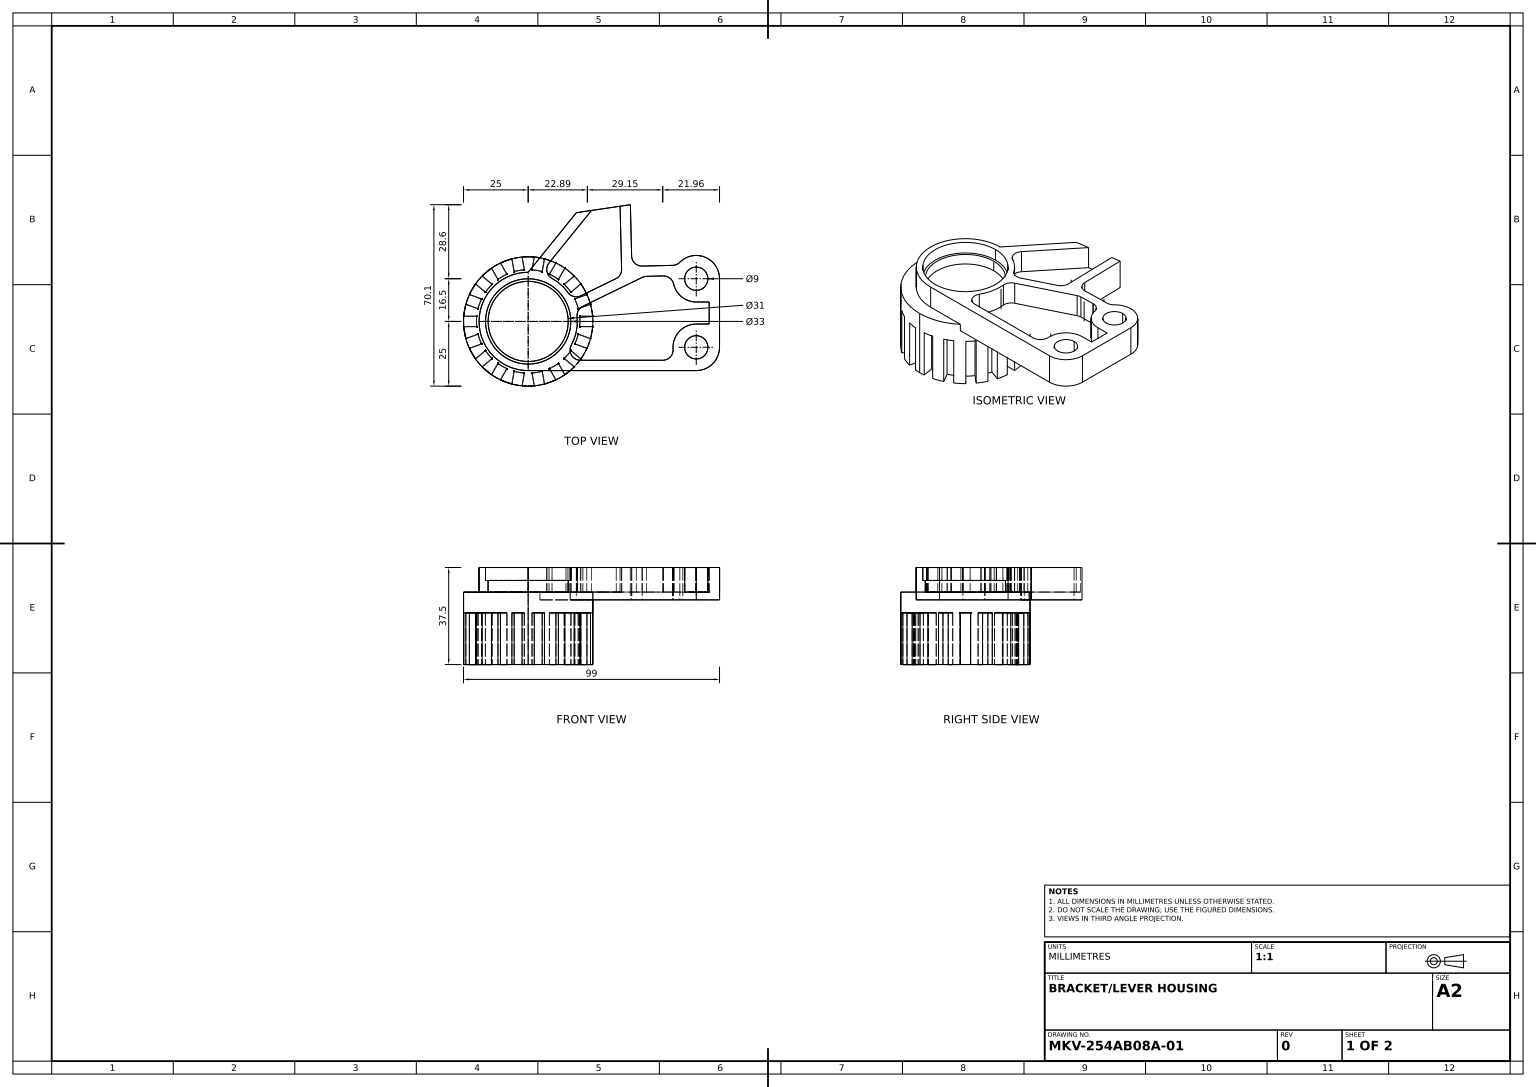
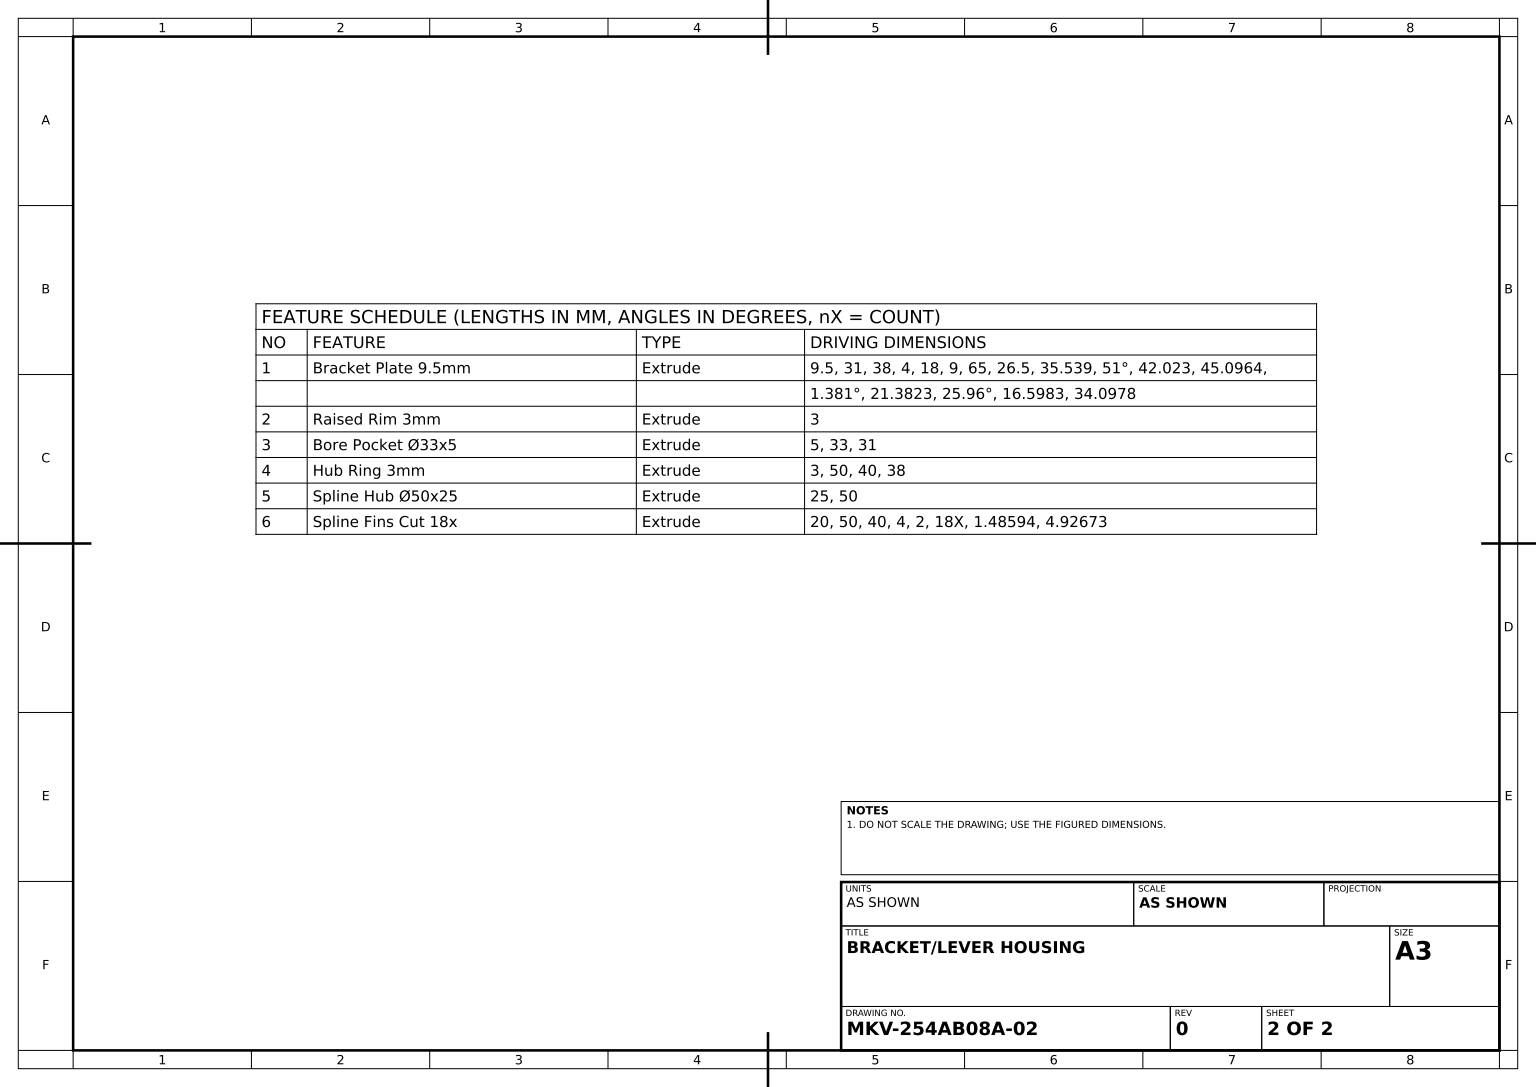
solid
v1 (65,0,14.5)
v2 (65,0,5.5)
e1 v1 v2 CIRCLE(AX(P(65,0,10),D(0,1,0),D(0,0,1)),4.5)
v3 (65,9.5,14.5)
e2 v3 v1 LINE
v4 (65,9.5,5.5)
e3 v3 v4 CIRCLE(AX(P(65,9.5,10),D(0,1,0),D(0,0,1)),4.5)
e4 v4 v2 LINE
face CYL(AX(P(65,9.5,10),D(0,-1,0),D(0,0,-1)),4.5) rev [-e1 -e2 e3 e4]
v5 (15.376876,9.5,-11.160273)
v6 (20.364842,9.5,-9.913285)
e5 v5 v6 CIRCLE(AX(P(18.614113,9.5,-13.509804),D(0,1,0),D(0,0,1)),4)
v7 (20.364842,0,-9.913285)
e6 v6 v7 LINE
v8 (15.376876,0,-11.160273)
e7 v8 v7 CIRCLE(AX(P(18.614113,0,-13.509804),D(0,1,0),D(0,0,1)),4)
e8 v5 v8 LINE
face CYL(AX(P(18.614113,9.5,-13.509804),D(0,-1,0),D(0,0,-1)),4) rev [e5 e6 -e7 -e8]
v9 (-19.899749,-28,-2)
v10 (-24.919872,-28,-2)
e9 v9 v10 LINE
v11 (-19.899749,-8,-2)
e10 v11 v9 LINE
v12 (-24.919872,-8,-2)
e11 v11 v12 LINE
e12 v12 v10 LINE
face PLANE(AX(P(0,-8,-2),D(0,0,1),D(1,0,0))) [-e9 -e10 e11 e12]
v13 (-1.48594,-8,19.944723)
v14 (-5.425171,-8,19.25013)
e13 v13 v14 CIRCLE(AX(P(0,-8,0),D(0,-1,0),D(0,0,-1)),20)
v15 (-5.425171,-28,19.25013)
e14 v14 v15 LINE
v16 (-1.48594,-28,19.944723)
e15 v16 v15 CIRCLE(AX(P(0,-28,0),D(0,-1,0),D(0,0,-1)),20)
e16 v13 v16 LINE
face CYL(AX(P(0,-8,0),D(0,-1,0),D(0,0,-1)),20) [e13 e14 -e15 -e16]
v17 (74,-3,-16.5)
v18 (74,-3,10)
e17 v17 v18 LINE
v19 (74,9.5,-16.5)
e18 v19 v17 LINE
v20 (74,9.5,10)
e19 v19 v20 LINE
e20 v20 v18 LINE
face PLANE(AX(P(74,9.5,0),D(1,0,0),D(0,0,-1))) [-e17 -e18 e19 e20]
v21 (-13.958517,-8,-14.323401)
v22 (-13.958517,-28,-14.323401)
e21 v21 v22 LINE
v23 (-16.529667,-28,-11.259223)
e22 v23 v22 CIRCLE(AX(P(0,-28,0),D(0,-1,0),D(0,0,-1)),20)
v24 (-16.529667,-8,-11.259223)
e23 v24 v23 LINE
e24 v24 v21 CIRCLE(AX(P(0,-8,0),D(0,-1,0),D(0,0,-1)),20)
face CYL(AX(P(0,-8,0),D(0,-1,0),D(0,0,-1)),20) [e21 -e22 -e23 e24]
v25 (52.236092,9.5,-17.577388)
v26 (52.236092,0,-17.577388)
e25 v25 v26 LINE
v27 (45.755023,9.5,-17.421109)
e26 v27 v25 LINE
v28 (45.755023,0,-17.421109)
e27 v27 v28 LINE
e28 v28 v26 LINE
face PLANE(AX(P(-0.393246,9.5,-16.308326),D(-0.024106198,0,-0.999709403),D(-0.999709403,0,0.024106198))) rev [-e25 -e26 e27 e28]
v29 (44.100719,9.5,-17.01879)
e29 v29 v27 CIRCLE(AX(P(45.851448,9.5,-13.422271),D(0,-1,0),D(0,0,1)),4)
v30 (44.100719,0,-17.01879)
e30 v29 v30 LINE
e31 v30 v28 CIRCLE(AX(P(45.851448,0,-13.422271),D(0,-1,0),D(0,0,1)),4)
face CYL(AX(P(45.851448,9.5,-13.422271),D(0,-1,0),D(0,0,-1)),4) rev [-e27 -e29 e30 e31]
v31 (36.125792,9.5,-20.175466)
v32 (36.125792,0,-20.175466)
e32 v31 v32 LINE
v33 (35.539017,9.5,-44.50962)
e33 v33 v31 LINE
v34 (35.539017,0,-44.50962)
e34 v33 v34 LINE
e35 v34 v32 LINE
face PLANE(AX(P(36.591011,9.5,-0.882327),D(0.999709403,0,-0.024106198),D(-0.024106198,0,-0.999709403))) rev [-e32 -e33 e34 e35]
v35 (11.681925,-8,-16.233688)
v36 (11.681925,-28,-16.233688)
e36 v35 v36 LINE
v37 (14.191987,-8,-20.581242)
e37 v35 v37 LINE
v38 (14.191987,-28,-20.581242)
e38 v37 v38 LINE
e39 v36 v38 LINE
face PLANE(AX(P(1.732051,-8,1),D(-0.866025404,0,-0.5),D(-0.5,0,0.866025404))) [-e36 e37 e38 -e39]
v39 (-17.804154,-8,-17.550274)
e40 v21 v39 LINE
v40 (-17.804154,-28,-17.550274)
e41 v39 v40 LINE
e42 v22 v40 LINE
face PLANE(AX(P(1.285575,-8,-1.532089),D(-0.64278761,0,0.766044443),D(0.766044443,0,0.64278761))) [-e21 e40 e41 -e42]
v41 (0,9.5,16.5)
v42 (0,9.5,-16.5)
e43 v41 v42 CIRCLE(AX(P(0,9.5,0),D(0,1,0),D(0,0,1)),16.5)
v43 (0,4.5,-16.5)
e44 v43 v42 LINE
v44 (0,4.5,16.5)
e45 v44 v43 CIRCLE(AX(P(0,4.5,0),D(0,1,0),D(0,0,1)),16.5)
e46 v44 v41 LINE
face CYL(AX(P(0,4.5,0),D(0,1,0),D(0,0,1)),16.5) rev [e43 -e44 -e45 e46]
v45 (1.48594,-8,-19.944723)
v46 (2.357675,-8,-24.888579)
e47 v45 v46 LINE
v47 (6.296906,-8,-24.193986)
e48 v46 v47 CIRCLE(AX(P(0,-8,0),D(0,-1,0),D(0,0,-1)),25)
v48 (5.425171,-8,-19.25013)
e49 v48 v47 LINE
e50 v45 v48 CIRCLE(AX(P(0,-8,0),D(0,-1,0),D(0,0,-1)),20)
face PLANE(AX(P(0,-8,0),D(0,-1,0),D(0,0,-1))) [e47 e48 -e49 -e50]
v49 (58.617258,9.5,-22.845125)
v50 (55.876909,9.5,-21.666343)
e51 v49 v50 CIRCLE(AX(P(55.780484,9.5,-25.66518),D(0,-1,0),D(0,0,1)),4)
v51 (58.617258,-3,-22.845125)
e52 v49 v51 LINE
v52 (55.876909,-3,-21.666343)
e53 v52 v51 CIRCLE(AX(P(55.780484,-3,-25.66518),D(0,1,0),D(0,0,-1)),4)
e54 v50 v52 LINE
face CYL(AX(P(55.780484,9.5,-25.66518),D(0,-1,0),D(0,0,-1)),4) rev [-e51 e52 -e53 -e54]
v53 (56.026667,9.5,10.692308)
v54 (56.026667,0,10.692308)
e55 v53 v54 LINE
v55 (65,9.5,1)
e56 v55 v53 CIRCLE(AX(P(65,9.5,10),D(0,1,0),D(0,0,1)),9)
v56 (65,0,1)
e57 v55 v56 LINE
e58 v56 v54 CIRCLE(AX(P(65,0,10),D(0,1,0),D(0,0,1)),9)
face CYL(AX(P(65,9.5,10),D(0,-1,0),D(0,0,-1)),9) [-e55 -e56 e57 e58]
v57 (-2.357675,-28,24.888579)
e59 v16 v57 LINE
v58 (-2.357675,-8,24.888579)
e60 v58 v57 LINE
e61 v13 v58 LINE
face PLANE(AX(P(1.969616,-8,0.347296),D(0.984807753,0,0.173648178),D(0.173648178,0,-0.984807753))) rev [e16 e59 -e60 -e61]
v59 (65,9.5,19)
v60 (65,-3,19)
e62 v59 v60 LINE
e63 v18 v60 CIRCLE(AX(P(65,-3,10),D(0,-1,0),D(0,0,-1)),9)
e64 v59 v20 CIRCLE(AX(P(65,9.5,10),D(0,1,0),D(0,0,1)),9)
face CYL(AX(P(65,9.5,10),D(0,-1,0),D(0,0,-1)),9) [e62 -e63 -e20 -e64]
v61 (19.899749,-8,2)
v62 (19.899749,-28,2)
e65 v61 v62 LINE
v63 (24.919872,-8,2)
e66 v61 v63 LINE
v64 (24.919872,-28,2)
e67 v63 v64 LINE
e68 v62 v64 LINE
face PLANE(AX(P(0,-8,2),D(0,0,-1),D(-1,0,0))) [-e65 e66 e67 -e68]
v65 (65,-3,-25.5)
e69 v65 v17 CIRCLE(AX(P(65,-3,-16.5),D(0,-1,0),D(0,0,-1)),9)
v66 (65,9.5,-25.5)
e70 v66 v65 LINE
e71 v19 v66 CIRCLE(AX(P(65,9.5,-16.5),D(0,1,0),D(0,0,1)),9)
face CYL(AX(P(65,9.5,-16.5),D(0,-1,0),D(0,0,-1)),9) [e18 -e69 -e70 -e71]
v67 (-18.015607,-8,8.6855)
v68 (-19.383687,-8,4.92673)
e72 v67 v68 CIRCLE(AX(P(0,-8,0),D(0,-1,0),D(0,0,-1)),20)
v69 (-22.732979,-8,10.402483)
e73 v67 v69 LINE
v70 (-24.10106,-8,6.643713)
e74 v69 v70 CIRCLE(AX(P(0,-8,0),D(0,-1,0),D(0,0,-1)),25)
e75 v68 v70 LINE
face PLANE(AX(P(0,-8,0),D(0,-1,0),D(0,0,-1))) [-e72 e73 e74 -e75]
v71 (-19.383687,-8,-4.92673)
v72 (-24.10106,-8,-6.643713)
e76 v71 v72 LINE
v73 (-22.732979,-8,-10.402483)
e77 v72 v73 CIRCLE(AX(P(0,-8,0),D(0,-1,0),D(0,0,-1)),25)
v74 (-18.015607,-8,-8.6855)
e78 v74 v73 LINE
e79 v71 v74 CIRCLE(AX(P(0,-8,0),D(0,-1,0),D(0,0,-1)),20)
face PLANE(AX(P(0,-8,0),D(0,-1,0),D(0,0,-1))) [e76 e77 -e78 -e79]
v75 (19.899749,-8,-2)
v76 (24.919872,-8,-2)
e80 v75 v76 LINE
e81 v76 v63 CIRCLE(AX(P(0,-8,0),D(0,-1,0),D(0,0,-1)),25)
e82 v75 v61 CIRCLE(AX(P(0,-8,0),D(0,-1,0),D(0,0,-1)),20)
face PLANE(AX(P(0,-8,0),D(0,-1,0),D(0,0,-1))) [e80 e81 -e66 -e82]
v77 (-13.958517,-8,14.323401)
v78 (-17.804154,-8,17.550274)
e83 v77 v78 LINE
v79 (-20.375304,-8,14.486096)
e84 v78 v79 CIRCLE(AX(P(0,-8,0),D(0,-1,0),D(0,0,-1)),25)
v80 (-16.529667,-8,11.259223)
e85 v80 v79 LINE
e86 v77 v80 CIRCLE(AX(P(0,-8,0),D(0,-1,0),D(0,0,-1)),20)
face PLANE(AX(P(0,-8,0),D(0,-1,0),D(0,0,-1))) [e83 e84 -e85 -e86]
v81 (-19.383687,-28,-4.92673)
v82 (-24.10106,-28,-6.643713)
e87 v81 v82 LINE
e88 v72 v82 LINE
e89 v71 v81 LINE
face PLANE(AX(P(-0.68404,-8,1.879385),D(-0.342020143,0,0.939692621),D(0.939692621,0,0.342020143))) rev [e87 -e88 -e76 e89]
v83 (-24.10106,-28,6.643713)
e90 v70 v83 LINE
v84 (-19.383687,-28,4.92673)
e91 v84 v83 LINE
e92 v68 v84 LINE
face PLANE(AX(P(-0.68404,-8,-1.879385),D(0.342020143,0,0.939692621),D(0.939692621,0,-0.342020143))) [e90 -e91 -e92 e75]
v85 (-22.732979,-28,10.402483)
e93 v69 v85 LINE
v86 (-18.015607,-28,8.6855)
e94 v67 v86 LINE
e95 v86 v85 LINE
face PLANE(AX(P(0.68404,-8,1.879385),D(0.342020143,0,0.939692621),D(0.939692621,0,-0.342020143))) rev [-e93 -e73 e94 e95]
v87 (20.19901,0,15)
v88 (52.038519,0,15)
e96 v87 v88 LINE
e97 v54 v88 CIRCLE(AX(P(52.038519,0,11),D(0,-1,0),D(0,0,1)),4)
v89 (70,0,1)
e98 v89 v56 LINE
v90 (70,0,-7.5)
e99 v90 v89 LINE
v91 (65,0,-7.5)
e100 v91 v90 LINE
v92 (56.230204,0,-14.477458)
e101 v92 v91 CIRCLE(AX(P(65,0,-16.5),D(0,1,0),D(0,0,1)),9)
v93 (52.332517,0,-17.578551)
e102 v93 v92 CIRCLE(AX(P(52.332517,0,-13.578551),D(0,-1,0),D(0,0,1)),4)
e103 v26 v93 CIRCLE(AX(P(52.332517,0,-13.578551),D(0,-1,0),D(0,0,1)),4)
v94 (21.139435,0,-5.841598)
e104 v94 v30 LINE
v95 (18.909266,0,-1.854631)
e105 v94 v95 CIRCLE(AX(P(22.890164,0,-2.245079),D(0,1,0),D(0,0,1)),4)
v96 (16.686139,0,9.086957)
e106 v96 v95 CIRCLE(AX(P(0,0,0),D(0,1,0),D(0,0,1)),19)
e107 v96 v87 CIRCLE(AX(P(20.19901,0,11),D(0,1,0),D(0,0,1)),4)
face PLANE(AX(P(0,0,0),D(0,-1,0),D(0,0,-1))) rev [e96 -e97 -e58 -e98 -e99 -e100 -e101 -e102 -e103 -e28 -e31 -e104 e105 -e106 e107]
v97 (21.139435,9.5,-5.841598)
e108 v97 v94 LINE
v98 (18.909266,9.5,-1.854631)
e109 v97 v98 CIRCLE(AX(P(22.890164,9.5,-2.245079),D(0,1,0),D(0,0,1)),4)
e110 v98 v95 LINE
face CYL(AX(P(22.890164,9.5,-2.245079),D(0,-1,0),D(0,0,-1)),4) rev [-e105 -e108 e109 e110]
v99 (20.375304,-8,-14.486096)
v100 (20.375304,-28,-14.486096)
e111 v99 v100 LINE
v101 (16.529667,-28,-11.259223)
e112 v101 v100 LINE
v102 (16.529667,-8,-11.259223)
e113 v102 v101 LINE
e114 v102 v99 LINE
face PLANE(AX(P(1.285575,-8,1.532089),D(-0.64278761,0,-0.766044443),D(-0.766044443,0,0.64278761))) [e111 -e112 -e113 e114]
v103 (65,9.5,-12)
v104 (65,0,-12)
e115 v103 v104 LINE
v105 (65,9.5,-21)
e116 v103 v105 CIRCLE(AX(P(65,9.5,-16.5),D(0,1,0),D(0,0,1)),4.5)
v106 (65,0,-21)
e117 v105 v106 LINE
e118 v104 v106 CIRCLE(AX(P(65,0,-16.5),D(0,1,0),D(0,0,1)),4.5)
face CYL(AX(P(65,9.5,-16.5),D(0,-1,0),D(0,0,-1)),4.5) rev [-e115 e116 e117 -e118]
e119 v86 v84 CIRCLE(AX(P(0,-28,0),D(0,-1,0),D(0,0,-1)),20)
face CYL(AX(P(0,-8,0),D(0,-1,0),D(0,0,-1)),20) [e92 -e119 -e94 e72]
v107 (-6.296906,-8,24.193986)
e120 v58 v107 CIRCLE(AX(P(0,-8,0),D(0,-1,0),D(0,0,-1)),25)
e121 v14 v107 LINE
face PLANE(AX(P(0,-8,0),D(0,-1,0),D(0,0,-1))) [e120 -e121 -e13 e61]
v108 (8.217824,-28,-18.233688)
v109 (10.727885,-28,-22.581242)
e122 v108 v109 LINE
v110 (10.727885,-8,-22.581242)
e123 v110 v109 LINE
v111 (8.217824,-8,-18.233688)
e124 v111 v110 LINE
e125 v111 v108 LINE
face PLANE(AX(P(-1.732051,-8,-1),D(-0.866025404,0,-0.5),D(-0.5,0,0.866025404))) rev [e122 -e123 -e124 e125]
v112 (-6.296906,-8,-24.193986)
v113 (-2.357675,-8,-24.888579)
e126 v112 v113 CIRCLE(AX(P(0,-8,0),D(0,-1,0),D(0,0,-1)),25)
v114 (-1.48594,-8,-19.944723)
e127 v114 v113 LINE
v115 (-5.425171,-8,-19.25013)
e128 v115 v114 CIRCLE(AX(P(0,-8,0),D(0,-1,0),D(0,0,-1)),20)
e129 v115 v112 LINE
face PLANE(AX(P(0,-8,0),D(0,-1,0),D(0,0,-1))) [e126 -e127 -e128 e129]
v116 (5.425171,-8,19.25013)
v117 (5.425171,-28,19.25013)
e130 v116 v117 LINE
v118 (1.48594,-8,19.944723)
e131 v116 v118 CIRCLE(AX(P(0,-8,0),D(0,-1,0),D(0,0,-1)),20)
v119 (1.48594,-28,19.944723)
e132 v118 v119 LINE
e133 v117 v119 CIRCLE(AX(P(0,-28,0),D(0,-1,0),D(0,0,-1)),20)
face CYL(AX(P(0,-8,0),D(0,-1,0),D(0,0,-1)),20) [-e130 e131 e132 -e133]
v120 (-19.899749,-8,2)
v121 (-19.899749,-28,2)
e134 v120 v121 LINE
e135 v120 v11 CIRCLE(AX(P(0,-8,0),D(0,-1,0),D(0,0,-1)),20)
e136 v121 v9 CIRCLE(AX(P(0,-28,0),D(0,-1,0),D(0,0,-1)),20)
face CYL(AX(P(0,-8,0),D(0,-1,0),D(0,0,-1)),20) [-e134 e135 e10 -e136]
e137 v106 v104 CIRCLE(AX(P(65,0,-16.5),D(0,1,0),D(0,0,1)),4.5)
face PLANE(AX(P(0,0,0),D(0,-1,0),D(0,0,-1))) rev [e118 e137]
v122 (52.332517,9.5,-17.578551)
e138 v122 v93 LINE
e139 v25 v122 CIRCLE(AX(P(52.332517,9.5,-13.578551),D(0,-1,0),D(0,0,1)),4)
face CYL(AX(P(52.332517,9.5,-13.578551),D(0,-1,0),D(0,0,-1)),4) rev [-e138 -e139 e25 e103]
v123 (-1.48594,-28,-19.944723)
v124 (-2.357675,-28,-24.888579)
e140 v123 v124 LINE
e141 v114 v123 LINE
e142 v113 v124 LINE
face PLANE(AX(P(1.969616,-8,-0.347296),D(-0.984807753,0,0.173648178),D(0.173648178,0,0.984807753))) [-e140 -e141 e127 e142]
v125 (34.097824,0,-16.598284)
e143 v32 v125 CIRCLE(AX(P(32.126954,0,-20.079042),D(0,-1,0),D(0,0,1)),4)
v126 (34.097824,9.5,-16.598284)
e144 v126 v125 LINE
e145 v31 v126 CIRCLE(AX(P(32.126954,9.5,-20.079042),D(0,-1,0),D(0,0,1)),4)
face CYL(AX(P(32.126954,9.5,-20.079042),D(0,-1,0),D(0,0,-1)),4) rev [e32 e143 -e144 -e145]
v127 (-10.727885,-8,-22.581242)
v128 (-10.727885,-28,-22.581242)
e146 v127 v128 LINE
v129 (-8.217824,-28,-18.233688)
e147 v129 v128 LINE
v130 (-8.217824,-8,-18.233688)
e148 v130 v129 LINE
e149 v130 v127 LINE
face PLANE(AX(P(1.732051,-8,-1),D(-0.866025404,0,0.5),D(0.5,0,0.866025404))) [e146 -e147 -e148 e149]
v131 (-22.732979,-28,-10.402483)
e150 v73 v131 LINE
e151 v10 v82 CIRCLE(AX(P(0,-28,0),D(0,-1,0),D(0,0,-1)),25)
v132 (-24.919872,-8,2)
e152 v132 v12 CIRCLE(AX(P(0,-8,0),D(0,-1,0),D(0,0,-1)),25)
v133 (-24.919872,-28,2)
e153 v132 v133 LINE
e154 v83 v133 CIRCLE(AX(P(0,-28,0),D(0,-1,0),D(0,0,-1)),25)
v134 (-20.375304,-28,14.486096)
e155 v134 v85 CIRCLE(AX(P(0,-28,0),D(0,-1,0),D(0,0,-1)),25)
e156 v79 v134 LINE
v135 (-17.804154,-28,17.550274)
e157 v78 v135 LINE
v136 (-14.191987,-28,20.581242)
e158 v136 v135 CIRCLE(AX(P(0,-28,0),D(0,-1,0),D(0,0,-1)),25)
v137 (-14.191987,-8,20.581242)
e159 v137 v136 LINE
v138 (-10.727885,-8,22.581242)
e160 v138 v137 CIRCLE(AX(P(0,-8,0),D(0,-1,0),D(0,0,-1)),25)
v139 (-10.727885,-28,22.581242)
e161 v138 v139 LINE
v140 (-6.296906,-28,24.193986)
e162 v140 v139 CIRCLE(AX(P(0,-28,0),D(0,-1,0),D(0,0,-1)),25)
e163 v107 v140 LINE
v141 (0,-28,25)
e164 v141 v57 CIRCLE(AX(P(0,-28,0),D(0,-1,0),D(0,0,-1)),25)
v142 (0,0,25)
e165 v142 v141 LINE
v143 (0,0,-25)
e166 v142 v143 CIRCLE(AX(P(0,0,0),D(0,-1,0),D(0,0,-1)),25)
v144 (0,-28,-25)
e167 v143 v144 LINE
e168 v124 v144 CIRCLE(AX(P(0,-28,0),D(0,-1,0),D(0,0,-1)),25)
v145 (-6.296906,-28,-24.193986)
e169 v112 v145 LINE
e170 v128 v145 CIRCLE(AX(P(0,-28,0),D(0,-1,0),D(0,0,-1)),25)
v146 (-14.191987,-8,-20.581242)
e171 v146 v127 CIRCLE(AX(P(0,-8,0),D(0,-1,0),D(0,0,-1)),25)
v147 (-14.191987,-28,-20.581242)
e172 v146 v147 LINE
e173 v40 v147 CIRCLE(AX(P(0,-28,0),D(0,-1,0),D(0,0,-1)),25)
v148 (-20.375304,-8,-14.486096)
e174 v148 v39 CIRCLE(AX(P(0,-8,0),D(0,-1,0),D(0,0,-1)),25)
v149 (-20.375304,-28,-14.486096)
e175 v148 v149 LINE
e176 v131 v149 CIRCLE(AX(P(0,-28,0),D(0,-1,0),D(0,0,-1)),25)
face CYL(AX(P(0,0,0),D(0,-1,0),D(0,0,-1)),25) [-e150 -e77 e88 -e151 -e12 -e152 e153 -e154 -e90 -e74 e93 -e155 -e156 -e84 e157 -e158 -e159 -e160 e161 -e162 -e163 -e120 e60 -e164 -e165 e166 e167 -e168 -e142 -e126 e169 -e170 -e146 -e171 e172 -e173 -e41 -e174 e175 -e176]
e177 v23 v149 LINE
e178 v24 v148 LINE
face PLANE(AX(P(-1.285575,-8,1.532089),D(-0.64278761,0,0.766044443),D(0.766044443,0,0.64278761))) rev [e177 -e175 -e178 e23]
v150 (8.217824,-8,18.233688)
v151 (8.217824,-28,18.233688)
e179 v150 v151 LINE
v152 (10.727885,-8,22.581242)
e180 v150 v152 LINE
v153 (10.727885,-28,22.581242)
e181 v152 v153 LINE
e182 v151 v153 LINE
face PLANE(AX(P(-1.732051,-8,1),D(0.866025404,0,-0.5),D(-0.5,0,-0.866025404))) [-e179 e180 e181 -e182]
v154 (19.383687,-28,4.92673)
v155 (24.10106,-28,6.643713)
e183 v154 v155 LINE
v156 (24.10106,-8,6.643713)
e184 v156 v155 LINE
v157 (19.383687,-8,4.92673)
e185 v157 v156 LINE
e186 v157 v154 LINE
face PLANE(AX(P(0.68404,-8,-1.879385),D(0.342020143,0,-0.939692621),D(-0.939692621,0,-0.342020143))) rev [e183 -e184 -e185 e186]
e187 v120 v132 LINE
face PLANE(AX(P(0,-8,0),D(0,-1,0),D(0,0,-1))) [e187 e152 -e11 -e135]
v158 (18.015607,-28,-8.6855)
v159 (19.383687,-28,-4.92673)
e188 v158 v159 CIRCLE(AX(P(0,-28,0),D(0,-1,0),D(0,0,-1)),20)
v160 (18.015607,-8,-8.6855)
e189 v160 v158 LINE
v161 (19.383687,-8,-4.92673)
e190 v160 v161 CIRCLE(AX(P(0,-8,0),D(0,-1,0),D(0,0,-1)),20)
e191 v161 v159 LINE
face CYL(AX(P(0,-8,0),D(0,-1,0),D(0,0,-1)),20) [-e188 -e189 e190 e191]
v162 (18.643636,9.5,-42.022974)
v163 (18.643636,-3,-42.022974)
e192 v162 v163 LINE
v164 (4.524413,-3,-24.587185)
e193 v164 v163 LINE
v165 (4.524413,0,-24.587185)
e194 v165 v164 LINE
v166 (0,0,-19)
e195 v166 v165 LINE
v167 (0,9.5,-19)
e196 v167 v166 LINE
e197 v167 v162 LINE
face PLANE(AX(P(-9.292402,9.5,-7.524839),D(-0.777145961,0,-0.629320391),D(-0.629320391,0,0.777145961))) [e192 -e193 -e194 -e195 -e196 e197]
v168 (11.681925,-8,16.233688)
v169 (14.191987,-8,20.581242)
e198 v168 v169 LINE
v170 (11.681925,-28,16.233688)
e199 v168 v170 LINE
v171 (14.191987,-28,20.581242)
e200 v170 v171 LINE
e201 v169 v171 LINE
face PLANE(AX(P(1.732051,-8,-1),D(0.866025404,0,-0.5),D(-0.5,0,-0.866025404))) rev [-e198 e199 e200 -e201]
v172 (44.099015,-3,-21.38234)
e202 v172 v52 LINE
v173 (44.099015,9.5,-21.38234)
e203 v173 v172 LINE
e204 v173 v50 LINE
face PLANE(AX(P(-0.489671,9.5,-20.307164),D(-0.024106198,0,-0.999709403),D(-0.999709403,0,0.024106198))) [-e202 -e203 e204 e54]
v174 (52.038519,9.5,15)
e205 v174 v88 LINE
e206 v53 v174 CIRCLE(AX(P(52.038519,9.5,11),D(0,-1,0),D(0,0,1)),4)
face CYL(AX(P(52.038519,9.5,11),D(0,-1,0),D(0,0,-1)),4) rev [e55 e97 -e205 -e206]
v175 (22.732979,-8,-10.402483)
v176 (22.732979,-28,-10.402483)
e207 v175 v176 LINE
e208 v160 v175 LINE
e209 v158 v176 LINE
face PLANE(AX(P(-0.68404,-8,-1.879385),D(-0.342020143,0,-0.939692621),D(-0.939692621,0,0.342020143))) rev [-e207 -e208 e189 e209]
v177 (2.357675,-8,24.888579)
v178 (2.357675,-28,24.888579)
e210 v177 v178 LINE
e211 v119 v178 LINE
e212 v118 v177 LINE
face PLANE(AX(P(-1.969616,-8,0.347296),D(0.984807753,0,-0.173648178),D(-0.173648178,0,-0.984807753))) [e210 -e211 -e132 e212]
e213 v121 v133 LINE
face PLANE(AX(P(0,-8,2),D(0,0,1),D(1,0,0))) rev [e213 -e153 -e187 e134]
v179 (39.52603,9.5,-45.096425)
v180 (39.52603,-3,-45.096425)
e214 v179 v180 LINE
e215 v163 v180 LINE
v181 (24.48712,9.5,-42.883012)
e216 v181 v162 LINE
v182 (24.48712,0,-42.883012)
e217 v181 v182 LINE
e218 v182 v34 LINE
e219 v179 v33 LINE
face PLANE(AX(P(-5.658478,9.5,-38.446211),D(0.145610435,0,0.989342004),D(0.989342004,0,-0.145610435))) rev [e214 -e215 -e192 -e216 e217 e218 -e34 -e219]
e220 v43 v44 CIRCLE(AX(P(0,4.5,0),D(0,1,0),D(0,0,1)),16.5)
e221 v42 v41 CIRCLE(AX(P(0,9.5,0),D(0,1,0),D(0,0,1)),16.5)
face CYL(AX(P(0,4.5,0),D(0,1,0),D(0,0,1)),16.5) rev [-e220 e44 e221 -e46]
v183 (56.230204,9.5,-14.477458)
e222 v183 v92 LINE
e223 v122 v183 CIRCLE(AX(P(52.332517,9.5,-13.578551),D(0,-1,0),D(0,0,1)),4)
face CYL(AX(P(52.332517,9.5,-13.578551),D(0,-1,0),D(0,0,-1)),4) rev [e138 e102 -e222 -e223]
v184 (-5.425171,-28,-19.25013)
e224 v115 v184 LINE
e225 v184 v145 LINE
face PLANE(AX(P(-1.969616,-8,0.347296),D(-0.984807753,0,0.173648178),D(0.173648178,0,0.984807753))) rev [-e169 -e129 e224 e225]
v185 (-11.681925,-8,-16.233688)
e226 v185 v146 LINE
v186 (-11.681925,-28,-16.233688)
e227 v185 v186 LINE
e228 v186 v147 LINE
face PLANE(AX(P(-1.732051,-8,1),D(-0.866025404,0,0.5),D(0.5,0,0.866025404))) rev [-e172 -e226 e227 e228]
v187 (40.003753,-3,-25.284753)
e229 v187 v172 CIRCLE(AX(P(44.002591,-3,-25.381178),D(0,1,0),D(0,0,-1)),4)
v188 (40.003753,9.5,-25.284753)
e230 v188 v187 LINE
e231 v173 v188 CIRCLE(AX(P(44.002591,9.5,-25.381178),D(0,-1,0),D(0,0,1)),4)
face CYL(AX(P(44.002591,9.5,-25.381178),D(0,-1,0),D(0,0,-1)),4) rev [-e229 -e230 -e231 e203]
e232 v6 v126 LINE
e233 v7 v125 LINE
face PLANE(AX(P(0,9.5,0),D(-0.43768221,0,-0.899129736),D(-0.899129736,0,0.43768221))) [-e6 e232 e144 -e233]
e234 v170 v151 CIRCLE(AX(P(0,-28,0),D(0,-1,0),D(0,0,-1)),20)
e235 v168 v150 CIRCLE(AX(P(0,-8,0),D(0,-1,0),D(0,0,-1)),20)
face CYL(AX(P(0,-8,0),D(0,-1,0),D(0,0,-1)),20) [-e234 -e199 e235 e179]
v189 (19.899749,-28,-2)
e236 v75 v189 LINE
e237 v189 v62 CIRCLE(AX(P(0,-28,0),D(0,-1,0),D(0,0,-1)),20)
face CYL(AX(P(0,-8,0),D(0,-1,0),D(0,0,-1)),20) [-e236 e82 e65 -e237]
v190 (-8.217824,-8,18.233688)
e238 v190 v138 LINE
v191 (-11.681925,-8,16.233688)
e239 v191 v137 LINE
e240 v190 v191 CIRCLE(AX(P(0,-8,0),D(0,-1,0),D(0,0,-1)),20)
face PLANE(AX(P(0,-8,0),D(0,-1,0),D(0,0,-1))) [e238 e160 -e239 -e240]
v192 (13.958517,-8,-14.323401)
e241 v192 v102 CIRCLE(AX(P(0,-8,0),D(0,-1,0),D(0,0,-1)),20)
v193 (17.804154,-8,-17.550274)
e242 v192 v193 LINE
e243 v193 v99 CIRCLE(AX(P(0,-8,0),D(0,-1,0),D(0,0,-1)),25)
face PLANE(AX(P(0,-8,0),D(0,-1,0),D(0,0,-1))) [-e241 e242 e243 -e114]
v194 (6.296906,-28,24.193986)
e244 v117 v194 LINE
v195 (6.296906,-8,24.193986)
e245 v195 v194 LINE
e246 v116 v195 LINE
face PLANE(AX(P(1.969616,-8,-0.347296),D(0.984807753,0,-0.173648178),D(-0.173648178,0,-0.984807753))) rev [e244 -e245 -e246 e130]
v196 (16.248077,0,19)
e247 v196 v142 CIRCLE(AX(P(0,0,0),D(0,-1,0),D(0,0,-1)),25)
e248 v178 v141 CIRCLE(AX(P(0,-28,0),D(0,-1,0),D(0,0,-1)),25)
e249 v195 v177 CIRCLE(AX(P(0,-8,0),D(0,-1,0),D(0,0,-1)),25)
e250 v153 v194 CIRCLE(AX(P(0,-28,0),D(0,-1,0),D(0,0,-1)),25)
e251 v169 v152 CIRCLE(AX(P(0,-8,0),D(0,-1,0),D(0,0,-1)),25)
v197 (17.804154,-28,17.550274)
e252 v197 v171 CIRCLE(AX(P(0,-28,0),D(0,-1,0),D(0,0,-1)),25)
v198 (17.804154,-8,17.550274)
e253 v198 v197 LINE
v199 (20.375304,-8,14.486096)
e254 v199 v198 CIRCLE(AX(P(0,-8,0),D(0,-1,0),D(0,0,-1)),25)
v200 (20.375304,-28,14.486096)
e255 v199 v200 LINE
v201 (22.732979,-28,10.402483)
e256 v201 v200 CIRCLE(AX(P(0,-28,0),D(0,-1,0),D(0,0,-1)),25)
v202 (22.732979,-8,10.402483)
e257 v202 v201 LINE
e258 v156 v202 CIRCLE(AX(P(0,-8,0),D(0,-1,0),D(0,0,-1)),25)
e259 v64 v155 CIRCLE(AX(P(0,-28,0),D(0,-1,0),D(0,0,-1)),25)
v203 (24.919872,-28,-2)
e260 v76 v203 LINE
v204 (24.10106,-28,-6.643713)
e261 v204 v203 CIRCLE(AX(P(0,-28,0),D(0,-1,0),D(0,0,-1)),25)
v205 (24.10106,-8,-6.643713)
e262 v205 v204 LINE
e263 v175 v205 CIRCLE(AX(P(0,-8,0),D(0,-1,0),D(0,0,-1)),25)
e264 v100 v176 CIRCLE(AX(P(0,-28,0),D(0,-1,0),D(0,0,-1)),25)
v206 (17.804154,-28,-17.550274)
e265 v193 v206 LINE
e266 v38 v206 CIRCLE(AX(P(0,-28,0),D(0,-1,0),D(0,0,-1)),25)
e267 v110 v37 CIRCLE(AX(P(0,-8,0),D(0,-1,0),D(0,0,-1)),25)
v207 (6.296906,-28,-24.193986)
e268 v207 v109 CIRCLE(AX(P(0,-28,0),D(0,-1,0),D(0,0,-1)),25)
e269 v47 v207 LINE
v208 (2.357675,-28,-24.888579)
e270 v46 v208 LINE
e271 v144 v208 CIRCLE(AX(P(0,-28,0),D(0,-1,0),D(0,0,-1)),25)
e272 v143 v165 CIRCLE(AX(P(0,0,0),D(0,-1,0),D(0,0,-1)),25)
v209 (16.248077,-3,19)
e273 v164 v209 CIRCLE(AX(P(0,-3,0),D(0,-1,0),D(0,0,-1)),25)
e274 v196 v209 LINE
face CYL(AX(P(0,0,0),D(0,-1,0),D(0,0,-1)),25) [e247 e165 -e248 -e210 -e249 e245 -e250 -e181 -e251 e201 -e252 -e253 -e254 e255 -e256 -e257 -e258 e184 -e259 -e67 -e81 e260 -e261 -e262 -e263 e207 -e264 -e111 -e243 e265 -e266 -e38 -e267 e123 -e268 -e269 -e48 e270 -e271 -e167 e272 e194 e273 -e274]
v210 (18.015607,-8,8.6855)
e275 v210 v202 LINE
e276 v157 v210 CIRCLE(AX(P(0,-8,0),D(0,-1,0),D(0,0,-1)),20)
face PLANE(AX(P(0,-8,0),D(0,-1,0),D(0,0,-1))) [-e275 -e276 e185 e258]
v211 (-16.529667,-28,11.259223)
e277 v211 v134 LINE
e278 v80 v211 LINE
face PLANE(AX(P(-1.285575,-8,-1.532089),D(0.64278761,0,0.766044443),D(0.766044443,0,-0.64278761))) [-e277 -e278 e85 e156]
e279 v51 v65 CIRCLE(AX(P(65,-3,-16.5),D(0,-1,0),D(0,0,-1)),9)
e280 v66 v49 CIRCLE(AX(P(65,9.5,-16.5),D(0,1,0),D(0,0,1)),9)
face CYL(AX(P(65,9.5,-16.5),D(0,-1,0),D(0,0,-1)),9) [e70 -e279 -e52 -e280]
face PLANE(AX(P(0,-8,0),D(0,-1,0),D(0,0,-1))) [e246 e249 -e212 -e131]
v212 (0,9.5,19)
v213 (0,0,19)
e281 v212 v213 LINE
e282 v167 v212 CIRCLE(AX(P(0,9.5,0),D(0,1,0),D(0,0,1)),19)
e283 v213 v166 CIRCLE(AX(P(0,0,0),D(0,-1,0),D(0,0,-1)),19)
face CYL(AX(P(0,9.5,0),D(0,-1,0),D(0,0,-1)),19) [-e281 -e282 e196 -e283]
e284 v161 v205 LINE
e285 v159 v204 LINE
face PLANE(AX(P(0.68404,-8,1.879385),D(-0.342020143,0,-0.939692621),D(-0.939692621,0,0.342020143))) [-e191 e284 e262 -e285]
v214 (20.19901,9.5,15)
e286 v214 v87 LINE
e287 v214 v174 LINE
face PLANE(AX(P(0,9.5,15),D(0,0,-1),D(-1,0,0))) [-e96 -e286 e287 e205]
v215 (13.958517,-8,14.323401)
e288 v215 v198 LINE
v216 (16.529667,-8,11.259223)
e289 v216 v215 CIRCLE(AX(P(0,-8,0),D(0,-1,0),D(0,0,-1)),20)
e290 v216 v199 LINE
face PLANE(AX(P(0,-8,0),D(0,-1,0),D(0,0,-1))) [e254 -e288 -e289 e290]
v217 (13.958517,-28,-14.323401)
e291 v192 v217 LINE
e292 v217 v206 LINE
face PLANE(AX(P(-1.285575,-8,-1.532089),D(-0.64278761,0,-0.766044443),D(-0.766044443,0,0.64278761))) rev [-e265 -e242 e291 e292]
e293 v105 v103 CIRCLE(AX(P(65,9.5,-16.5),D(0,1,0),D(0,0,1)),4.5)
face CYL(AX(P(65,9.5,-16.5),D(0,-1,0),D(0,0,-1)),4.5) rev [-e137 -e117 e293 e115]
e294 v60 v209 LINE
e295 v212 v59 LINE
e296 v196 v213 LINE
face PLANE(AX(P(0,9.5,19),D(0,0,-1),D(-1,0,0))) rev [e274 -e294 -e62 -e295 e281 -e296]
v218 (65,9.5,-7.5)
e297 v183 v218 CIRCLE(AX(P(65,9.5,-16.5),D(0,1,0),D(0,0,1)),9)
v219 (70,9.5,-7.5)
e298 v218 v219 LINE
v220 (70,9.5,1)
e299 v219 v220 LINE
e300 v220 v55 LINE
v221 (16.686139,9.5,9.086957)
e301 v221 v214 CIRCLE(AX(P(20.19901,9.5,11),D(0,1,0),D(0,0,1)),4)
e302 v221 v98 CIRCLE(AX(P(0,9.5,0),D(0,1,0),D(0,0,1)),19)
e303 v97 v29 LINE
e304 v179 v188 LINE
v222 (9.238381,9.5,-16.602781)
e305 v5 v222 CIRCLE(AX(P(0,9.5,0),D(0,1,0),D(0,0,1)),19)
v223 (8.074719,9.5,-22.615384)
e306 v223 v222 CIRCLE(AX(P(11.183303,9.5,-20.098103),D(0,1,0),D(0,0,1)),4)
e307 v223 v181 LINE
e308 v4 v3 CIRCLE(AX(P(65,9.5,10),D(0,1,0),D(0,0,1)),4.5)
face PLANE(AX(P(0,9.5,0),D(0,1,0),D(0,0,1))) [-e43 -e221] [e139 e223 e297 e298 e299 e300 e56 e206 -e287 -e301 e302 -e109 e303 e29 e26] [-e293 -e116] [e64 -e19 e71 e280 e51 -e204 e231 -e304 e219 e33 e145 -e232 -e5 e305 -e306 e307 e216 -e197 e282 e295] [-e3 -e308]
v224 (9.238381,0,-16.602781)
e309 v8 v224 CIRCLE(AX(P(0,0,0),D(0,1,0),D(0,0,1)),19)
e310 v222 v224 LINE
face CYL(AX(P(0,9.5,0),D(0,-1,0),D(0,0,-1)),19) [e309 -e310 -e305 e8]
v225 (-13.958517,-28,14.323401)
e311 v77 v225 LINE
e312 v225 v135 LINE
face PLANE(AX(P(1.285575,-8,1.532089),D(0.64278761,0,0.766044443),D(0.766044443,0,-0.64278761))) rev [-e83 e311 e312 -e157]
v226 (13.958517,-28,14.323401)
e313 v226 v197 LINE
e314 v215 v226 LINE
face PLANE(AX(P(-1.285575,-8,1.532089),D(0.64278761,0,-0.766044443),D(-0.766044443,0,-0.64278761))) [e253 -e313 -e314 e288]
face PLANE(AX(P(0,-8,0),D(0,-1,0),D(0,0,-1))) [-e190 e208 e263 -e284]
v227 (8.074719,0,-22.615384)
e315 v227 v182 LINE
e316 v227 v224 CIRCLE(AX(P(11.183303,0,-20.098103),D(0,1,0),D(0,0,1)),4)
face PLANE(AX(P(0,0,0),D(0,-1,0),D(0,0,-1))) rev [-e218 -e315 e316 -e309 e7 e233 -e143 -e35]
e317 v185 v130 CIRCLE(AX(P(0,-8,0),D(0,-1,0),D(0,0,-1)),20)
e318 v186 v129 CIRCLE(AX(P(0,-28,0),D(0,-1,0),D(0,0,-1)),20)
face CYL(AX(P(0,-8,0),D(0,-1,0),D(0,0,-1)),20) [-e227 e317 e148 -e318]
e319 v219 v90 LINE
e320 v218 v91 LINE
face PLANE(AX(P(0,9.5,-7.5),D(0,0,-1),D(-1,0,0))) rev [-e319 -e298 e320 e100]
e321 v217 v101 CIRCLE(AX(P(0,-28,0),D(0,-1,0),D(0,0,-1)),20)
face CYL(AX(P(0,-8,0),D(0,-1,0),D(0,0,-1)),20) [e113 -e321 -e291 e241]
v228 (1.48594,-28,-19.944723)
e322 v45 v228 LINE
e323 v228 v208 LINE
face PLANE(AX(P(-1.969616,-8,-0.347296),D(-0.984807753,0,-0.173648178),D(-0.173648178,0,0.984807753))) rev [e322 e323 -e270 -e47]
e324 v2 v1 CIRCLE(AX(P(65,0,10),D(0,1,0),D(0,0,1)),4.5)
face CYL(AX(P(65,9.5,10),D(0,-1,0),D(0,0,-1)),4.5) rev [-e324 -e4 e308 e2]
v229 (0,0,15.5)
v230 (0,0,-15.5)
e325 v229 v230 CIRCLE(AX(P(0,0,0),D(0,1,0),D(0,0,1)),15.5)
e326 v230 v229 CIRCLE(AX(P(0,0,0),D(0,1,0),D(0,0,1)),15.5)
face PLANE(AX(P(0,0,0),D(0,-1,0),D(0,0,-1))) rev [e325 e326]
e327 v180 v187 LINE
face PLANE(AX(P(40.589849,9.5,-0.978751),D(0.999709403,0,-0.024106198),D(-0.024106198,0,-0.999709403))) [e304 e230 -e327 -e214]
e328 v223 v227 LINE
face PLANE(AX(P(-6.183818,9.5,-5.007557),D(-0.777145961,0,-0.629320391),D(-0.629320391,0,0.777145961))) rev [-e307 e328 e315 -e217]
face PLANE(AX(P(0,0,0),D(0,-1,0),D(0,0,-1))) rev [e1 e324]
v231 (-8.217824,-28,18.233688)
e329 v190 v231 LINE
v232 (-11.681925,-28,16.233688)
e330 v191 v232 LINE
e331 v231 v232 CIRCLE(AX(P(0,-28,0),D(0,-1,0),D(0,0,-1)),20)
face CYL(AX(P(0,-8,0),D(0,-1,0),D(0,0,-1)),20) [-e329 e240 e330 -e331]
face CYL(AX(P(11.183303,9.5,-20.098103),D(0,-1,0),D(0,0,-1)),4) rev [e306 e310 -e316 -e328]
v233 (-18.015607,-28,-8.6855)
e332 v74 v233 LINE
e333 v81 v233 CIRCLE(AX(P(0,-28,0),D(0,-1,0),D(0,0,-1)),20)
face CYL(AX(P(0,-8,0),D(0,-1,0),D(0,0,-1)),20) [-e89 e79 e332 -e333]
face PLANE(AX(P(0,-8,0),D(0,-1,0),D(0,0,-1))) [e174 -e40 -e24 e178]
e334 v189 v203 LINE
face PLANE(AX(P(0,-8,-2),D(0,0,-1),D(-1,0,0))) rev [e236 e334 -e260 -e80]
v234 (0,4.5,-15.5)
e335 v234 v230 LINE
v235 (0,4.5,15.5)
e336 v235 v229 LINE
e337 v235 v234 CIRCLE(AX(P(0,4.5,0),D(0,1,0),D(0,0,1)),15.5)
face CYL(AX(P(0,9.5,0),D(0,-1,0),D(0,0,-1)),15.5) rev [e335 -e325 -e336 e337]
e338 v220 v89 LINE
face PLANE(AX(P(0,9.5,1),D(0,0,1),D(1,0,0))) rev [e338 e98 -e57 -e300]
e339 v111 v35 CIRCLE(AX(P(0,-8,0),D(0,-1,0),D(0,0,-1)),20)
face PLANE(AX(P(0,-8,0),D(0,-1,0),D(0,0,-1))) [-e37 -e339 e124 e267]
v236 (18.015607,-28,8.6855)
e340 v210 v236 LINE
e341 v154 v236 CIRCLE(AX(P(0,-28,0),D(0,-1,0),D(0,0,-1)),20)
face CYL(AX(P(0,-8,0),D(0,-1,0),D(0,0,-1)),20) [e276 e340 -e341 -e186]
v237 (5.425171,-28,-19.25013)
e342 v237 v207 LINE
e343 v48 v237 LINE
face PLANE(AX(P(1.969616,-8,0.347296),D(-0.984807753,0,-0.173648178),D(-0.173648178,0,0.984807753))) [e49 e269 -e342 -e343]
face PLANE(AX(P(0,0,0),D(0,-1,0),D(0,0,-1))) rev [e283 e195 -e272 -e166 -e247 e296]
e344 v184 v123 CIRCLE(AX(P(0,-28,0),D(0,-1,0),D(0,0,-1)),20)
face CYL(AX(P(0,-8,0),D(0,-1,0),D(0,0,-1)),20) [e128 e141 -e344 -e224]
v238 (16.529667,-28,11.259223)
e345 v238 v226 CIRCLE(AX(P(0,-28,0),D(0,-1,0),D(0,0,-1)),20)
e346 v216 v238 LINE
face CYL(AX(P(0,-8,0),D(0,-1,0),D(0,0,-1)),20) [e314 -e345 -e346 e289]
e347 v15 v140 LINE
face PLANE(AX(P(-1.969616,-8,-0.347296),D(0.984807753,0,0.173648178),D(0.173648178,0,-0.984807753))) [-e347 -e14 e121 e163]
face PLANE(AX(P(0,-8,0),D(0,-1,0),D(0,0,-1))) [e198 e251 -e180 -e235]
face PLANE(AX(P(1.750729,9.5,3.596519),D(-0.43768221,0,-0.899129736),D(-0.899129736,0,0.43768221))) rev [e104 -e30 -e303 e108]
e348 v232 v136 LINE
face PLANE(AX(P(-1.732051,-8,-1),D(0.866025404,0,0.5),D(0.5,0,-0.866025404))) [e159 -e348 -e330 e239]
e349 v236 v201 LINE
e350 v238 v200 LINE
e351 v231 v139 LINE
e352 v225 v211 CIRCLE(AX(P(0,-28,0),D(0,-1,0),D(0,0,-1)),20)
e353 v233 v131 LINE
e354 v228 v237 CIRCLE(AX(P(0,-28,0),D(0,-1,0),D(0,0,-1)),20)
e355 v108 v36 CIRCLE(AX(P(0,-28,0),D(0,-1,0),D(0,0,-1)),20)
face PLANE(AX(P(0,-28,0),D(0,-1,0),D(0,0,-1))) [e237 e68 e259 -e183 e341 e349 e256 -e350 e345 e313 e252 -e200 e234 e182 e250 -e244 e133 e211 e248 e164 -e59 e15 e347 e162 -e351 e331 e348 e158 -e312 e352 e277 e155 -e95 e119 e91 e154 -e213 e136 e9 e151 -e87 e333 e353 e176 -e177 e22 e42 e173 -e228 e318 e147 e170 -e225 e344 e140 e168 e271 -e323 e354 e342 e268 -e122 e355 e39 e266 -e292 e321 e112 e264 -e209 e188 e285 e261 -e334]
face PLANE(AX(P(0,-8,0),D(0,-1,0),D(0,0,-1))) [-e149 -e317 e226 e171]
face PLANE(AX(P(1.285575,-8,-1.532089),D(0.64278761,0,-0.766044443),D(-0.766044443,0,-0.64278761))) rev [e346 e350 -e255 -e290]
e356 v234 v235 CIRCLE(AX(P(0,4.5,0),D(0,1,0),D(0,0,1)),15.5)
face CYL(AX(P(0,9.5,0),D(0,-1,0),D(0,0,-1)),15.5) rev [e356 e336 -e326 -e335]
e357 v221 v96 LINE
face CYL(AX(P(20.19901,9.5,11),D(0,-1,0),D(0,0,-1)),4) rev [-e357 e301 e286 -e107]
face PLANE(AX(P(70,9.5,0),D(1,0,0),D(0,0,-1))) rev [e99 -e338 -e299 e319]
face CYL(AX(P(0,9.5,0),D(0,-1,0),D(0,0,-1)),19) [e357 e106 -e110 -e302]
face CYL(AX(P(0,-8,0),D(0,-1,0),D(0,0,-1)),20) [e278 -e352 -e311 e86]
face CYL(AX(P(0,-8,0),D(0,-1,0),D(0,0,-1)),20) [-e355 -e125 e339 e36]
face CYL(AX(P(0,-8,0),D(0,-1,0),D(0,0,-1)),20) [-e354 -e322 e50 e343]
face PLANE(AX(P(1.732051,-8,1),D(0.866025404,0,0.5),D(0.5,0,-0.866025404))) rev [e329 e351 -e161 -e238]
face CYL(AX(P(65,9.5,-16.5),D(0,-1,0),D(0,0,-1)),9) [-e320 -e297 e222 e101]
face PLANE(AX(P(0,-3,0),D(0,-1,0),D(0,0,-1))) [e53 e279 e69 e17 e63 e294 -e273 e193 e215 e327 e229 e202]
face PLANE(AX(P(-0.68404,-8,1.879385),D(0.342020143,0,-0.939692621),D(-0.939692621,0,-0.342020143))) [-e349 -e340 e275 e257]
face PLANE(AX(P(0.68404,-8,-1.879385),D(-0.342020143,0,0.939692621),D(0.939692621,0,0.342020143))) [-e353 -e332 e78 e150]
face PLANE(AX(P(0,4.5,0),D(0,1,0),D(0,0,1))) [e45 e220] [-e337 -e356]
